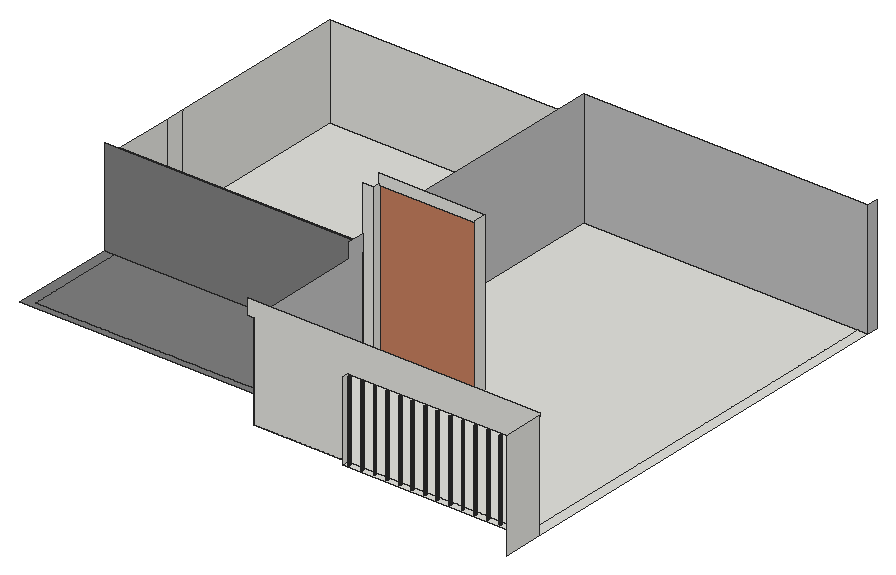
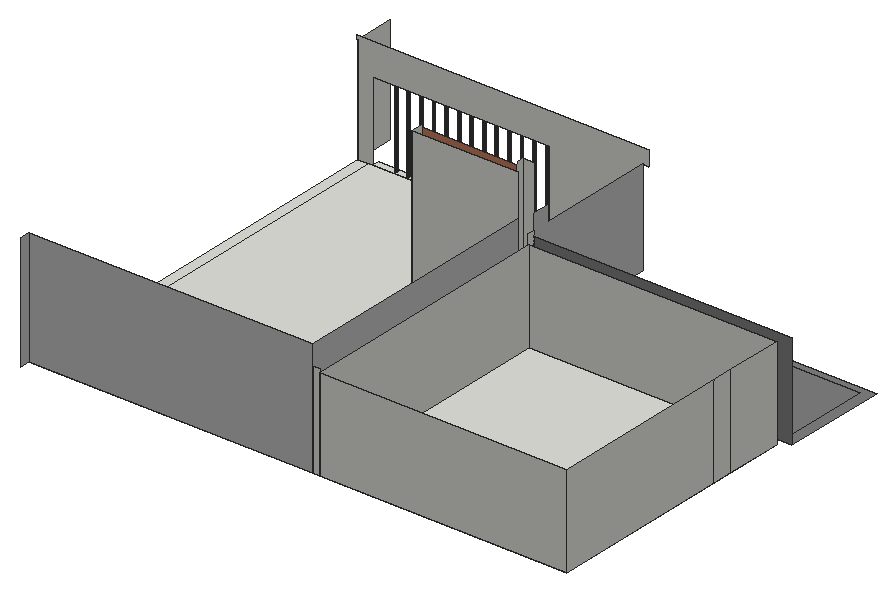
# SketchUp Ruby script. Lengths in inches.
U = 1.inch
M = Sketchup.active_model
def pt(a) = Geom::Point3d.new(a.map { |v| v * U })
def face(e, loops, mat)
  f = e.add_face(loops[0].map { |a| pt(a) })
  loops[1..].each { |l| e.add_face(l.map { |a| pt(a) }).erase! }
  f.material = f.back_material = mat if mat
  f
end
# faces: each face lists its corners as indices into pts; further lists are holes
def faces(e, pts, list, mat = nil) = list.each { |f| face(e, (f[0].is_a?(Array) ? f : [f]).map { |l| l.map { |i| pts[i] } }, mat) }
# xy, xz, yz: faces in a plane at the given z, y or x. An outline is a flat list of corners, or four numbers for a rectangle; further outlines are holes
def ring(l) = l.size == 4 ? [[l[0], l[1]], [l[2], l[1]], [l[2], l[3]], [l[0], l[3]]] : l.each_slice(2).to_a
def flat(e, list, mat, &to3) = list.each { |f| face(e, (f[0].is_a?(Array) ? f : [f]).map { |l| ring(l).map { |u, v| to3.(u, v) } }, mat) }
def xy(e, z, list, mat = nil) = flat(e, list, mat) { |x, y| [x, y, z] }
def xz(e, y, list, mat = nil) = flat(e, list, mat) { |x, z| [x, y, z] }
def yz(e, x, list, mat = nil) = flat(e, list, mat) { |y, z| [x, y, z] }
def lines(e, pts, list) = list.each { |a, b| e.add_line(pt(pts[a]), pt(pts[b])) }
# prism: a flat outline (further loops are holes) pulled along v
def prism(e, loops, v, mat = nil)
  f = face(e, loops, mat); d = Geom::Vector3d.new(v.map { |x| x * U })
  f.pushpull(f.normal.samedirection?(d) ? d.length : -d.length)
end
def box(e, o, s, mat = nil) = prism(e, [[o, [o[0] + s[0], o[1], o[2]], [o[0] + s[0], o[1] + s[1], o[2]], [o[0], o[1] + s[1], o[2]]]], [0, 0, s[2]], mat)
def at(x, y, z, deg = 0) = Geom::Transformation.translation(pt([x, y, z])) * Geom::Transformation.rotation(ORIGIN, Z_AXIS, deg.degrees)
def axes(o, x, y, z) = Geom::Transformation.new([*x, 0, *y, 0, *z, 0, *pt(o).to_a, 1])
def part(name) = M.definitions.add(name)
# library, detail: a bought-in or finely detailed component or shape, given as its bounding box
def library(name, o, s) = part(name).tap { |d| box(d.entities, o, s) }
def detail(e, o, s) = box(e.add_group.entities, o, s)
def put(e, d, t, mat = nil) = e.add_instance(d, t).tap { |i| i.material = mat if mat }
def group(e, t, mat = nil) = e.add_group.tap { |g| g.transformation = t; g.material = mat if mat }.entities
root = M.entities
M.materials.add("[0131_Silver]").color = [192, 192, 192]
M.materials.add("[0133_Gray]").color = [128, 128, 128]
M.materials.add("[0136_Charcoal]").color = [35, 35, 35]
M.materials.add("[Cladding Siding Tan]").color = [197, 126, 95]
xy(root,410,[[[329.48,44.6875,482.9375,50.6875],[333.11,46.6875,332.91,46.71,332.71,46.77,332.53,46.88,332.37,47.02,332.25,47.1875,332.16,47.38,332.12,47.58,332.12,47.79,332.16,48,332.25,48.1875,332.37,48.36,332.53,48.5,332.71,48.6,332.91,48.67,333.11,48.6875,333.32,48.67,333.52,48.6,333.7,48.5,333.86,48.36,333.98,48.1875,334.0625,48,334.11,47.79,334.11,47.58,334.0625,47.38,333.98,47.1875,333.86,47.02,333.7,46.88,333.52,46.77,333.32,46.71]],[333.11,46.6875,332.91,46.71,332.71,46.77,332.53,46.88,332.37,47.02,332.25,47.1875,332.16,47.38,332.12,47.58,332.12,47.79,332.16,48,332.25,48.1875,332.37,48.36,332.53,48.5,332.71,48.6,332.91,48.67,333.11,48.6875,333.32,48.67,333.52,48.6,333.7,48.5,333.86,48.36,333.98,48.1875,334.0625,48,334.11,47.79,334.11,47.58,334.0625,47.38,333.98,47.1875,333.86,47.02,333.7,46.88,333.52,46.77,333.32,46.71],[247.25,50.6875,486.875,50.6875,486.875,411,247.25,411,247.25,187,339.9375,187,339.9375,176.25,256.62,176.25,256.62,169.5,247.25,169.5],[486.875,50.6875,495.875,411],[247.25,169.5,256.62,176.25],
  [24.875,182.25,241.25,411]])
xy(root,410,[[15.875,84.25,241.25,84.25,241.25,90.25,24.875,90.25,24.875,176.25,15.875,176.25],[24.875,90.25,241.25,176.25]],"[0133_Gray]")
xz(root,50.6875,[[247.25,410,247.25,494,241.25,494,241.25,506.875,497.375,506.875,497.375,503.875,495.875,503.875,495.875,410,482.9375,410,482.9375,479,329.48,479,329.48,410]])
xz(root,169.5,[[247.25,410,256.62,547.1875]])
xz(root,176.25,[[15.875,410,241.25,494]],"[0133_Gray]")
xz(root,176.25,[[256.62,410,339.9375,545.23]],"[Cladding Siding Tan]")
xz(root,182.25,[[24.875,410,241.25,490.625]])
xz(root,187,[[247.25,410,339.9375,547.1875]])
xz(root,411,[[24.875,410,241.25,490.625],[241.25,410,247.25,494]])
xz(root,411,[[247.25,410,495.875,511]],"[0131_Silver]")
yz(root,24.875,[[182.25,410,233.22,490.625],[233.22,410,250.625,490.625],[250.625,410,411,490.625]])
yz(root,241.25,[[182.25,410,411,490.625]])
yz(root,247.25,[[169.5,410,176.25,494]])
yz(root,247.25,[[50.6875,410,169.5,410,169.5,507.4375,154.25,507.4375,154.25,494,50.6875,494],[187,410,411,511]],"[0131_Silver]")
yz(root,256.62,[[169.5,410,176.25,410,176.25,545.23,175.6875,545.23,175.6875,547.1875,169.5,547.1875]])
yz(root,329.48,[[44.6875,410,50.6875,479]])
yz(root,332.12,[[47.58,410,47.79,479]],"[0136_Charcoal]")
yz(root,334.11,[[47.58,410,47.79,479]],"[0136_Charcoal]")
yz(root,339.9375,[[176.25,410,187,410,187,547.1875,175.6875,547.1875,175.6875,545.23,176.25,545.23]])
yz(root,343.12,[[47.58,410,47.79,479]],"[0136_Charcoal]")
yz(root,345.11,[[47.58,410,47.79,479]],"[0136_Charcoal]")
yz(root,354.12,[[47.58,410,47.79,479]],"[0136_Charcoal]")
yz(root,356.11,[[47.58,410,47.79,479]],"[0136_Charcoal]")
yz(root,365.12,[[47.58,410,47.79,479]],"[0136_Charcoal]")
yz(root,367.11,[[47.58,410,47.79,479]],"[0136_Charcoal]")
yz(root,376.12,[[47.58,410,47.79,479]],"[0136_Charcoal]")
yz(root,378.11,[[47.58,410,47.79,479]],"[0136_Charcoal]")
yz(root,387.12,[[47.58,410,47.79,479]],"[0136_Charcoal]")
yz(root,389.11,[[47.58,410,47.79,479]],"[0136_Charcoal]")
yz(root,398.12,[[47.58,410,47.79,479]],"[0136_Charcoal]")
yz(root,400.11,[[47.58,410,47.79,479]],"[0136_Charcoal]")
yz(root,409.12,[[47.58,410,47.79,479]],"[0136_Charcoal]")
yz(root,411.11,[[47.58,410,47.79,479]],"[0136_Charcoal]")
yz(root,420.12,[[47.58,410,47.79,479]],"[0136_Charcoal]")
yz(root,422.11,[[47.58,410,47.79,479]],"[0136_Charcoal]")
yz(root,431.12,[[47.58,410,47.79,479]],"[0136_Charcoal]")
yz(root,433.11,[[47.58,410,47.79,479]],"[0136_Charcoal]")
yz(root,442.12,[[47.58,410,47.79,479]],"[0136_Charcoal]")
yz(root,444.11,[[47.58,410,47.79,479]],"[0136_Charcoal]")
yz(root,453.12,[[47.58,410,47.79,479]],"[0136_Charcoal]")
yz(root,455.11,[[47.58,410,47.79,479]],"[0136_Charcoal]")
yz(root,464.12,[[47.58,410,47.79,479]],"[0136_Charcoal]")
yz(root,466.11,[[47.58,410,47.79,479]],"[0136_Charcoal]")
yz(root,495.875,[[15.6875,410,50.6875,503.875]])
yz(root,495.875,[[411,410,420,511]],"[0131_Silver]")
p = [[332.71,46.77,410],[332.91,46.71,410],[332.91,46.71,479],[332.71,46.77,479],[333.11,46.6875,410],[333.11,46.6875,479],
  [333.32,46.71,410],[333.32,46.71,479],[333.52,46.77,410],[333.52,46.77,479],[343.71,46.77,410],[343.91,46.71,410],
  [343.91,46.71,479],[343.71,46.77,479],[344.11,46.6875,410],[344.11,46.6875,479],[344.32,46.71,410],[344.32,46.71,479],
  [344.52,46.77,410],[344.52,46.77,479],[354.71,46.77,410],[354.91,46.71,410],[354.91,46.71,479],[354.71,46.77,479],
  [355.11,46.6875,410],[355.11,46.6875,479],[355.32,46.71,410],[355.32,46.71,479],[355.52,46.77,410],[355.52,46.77,479],
  [365.71,46.77,410],[365.91,46.71,410],[365.91,46.71,479],[365.71,46.77,479],[366.11,46.6875,410],[366.11,46.6875,479],
  [366.32,46.71,410],[366.32,46.71,479],[366.52,46.77,410],[366.52,46.77,479],[376.71,46.77,410],[376.91,46.71,410],
  [376.91,46.71,479],[376.71,46.77,479],[377.11,46.6875,410],[377.11,46.6875,479],[377.32,46.71,410],[377.32,46.71,479],
  [377.52,46.77,410],[377.52,46.77,479],[387.71,46.77,410],[387.91,46.71,410],[387.91,46.71,479],[387.71,46.77,479],
  [388.11,46.6875,410],[388.11,46.6875,479],[388.32,46.71,410],[388.32,46.71,479],[388.52,46.77,410],[388.52,46.77,479],
  [398.71,46.77,410],[398.91,46.71,410],[398.91,46.71,479],[398.71,46.77,479],[399.11,46.6875,410],[399.11,46.6875,479],
  [399.32,46.71,410],[399.32,46.71,479],[399.52,46.77,410],[399.52,46.77,479],[409.71,46.77,410],[409.91,46.71,410],
  [409.91,46.71,479],[409.71,46.77,479],[410.11,46.6875,410],[410.11,46.6875,479],[410.32,46.71,410],[410.32,46.71,479],
  [410.52,46.77,410],[410.52,46.77,479],[420.71,46.77,410],[420.91,46.71,410],[420.91,46.71,479],[420.71,46.77,479],
  [421.11,46.6875,410],[421.11,46.6875,479],[421.32,46.71,410],[421.32,46.71,479],[421.52,46.77,410],[421.52,46.77,479],
  [431.71,46.77,410],[431.91,46.71,410],[431.91,46.71,479],[431.71,46.77,479],[432.11,46.6875,410],[432.11,46.6875,479],
  [432.32,46.71,410],[432.32,46.71,479],[432.52,46.77,410],[432.52,46.77,479],[442.71,46.77,410],[442.91,46.71,410],
  [442.91,46.71,479],[442.71,46.77,479],[443.11,46.6875,410],[443.11,46.6875,479],[443.32,46.71,410],[443.32,46.71,479],
  [443.52,46.77,410],[443.52,46.77,479],[453.71,46.77,410],[453.91,46.71,410],[453.91,46.71,479],[453.71,46.77,479],
  [454.11,46.6875,410],[454.11,46.6875,479],[454.32,46.71,410],[454.32,46.71,479],[454.52,46.77,410],[454.52,46.77,479],
  [464.71,46.77,410],[464.91,46.71,410],[464.91,46.71,479],[464.71,46.77,479],[465.11,46.6875,410],[465.11,46.6875,479],
  [465.32,46.71,410],[465.32,46.71,479],[465.52,46.77,410],[465.52,46.77,479],[332.53,46.88,410],[332.53,46.88,479],
  [333.7,46.88,410],[333.7,46.88,479],[343.53,46.88,410],[343.53,46.88,479],[344.7,46.88,410],[344.7,46.88,479],
  [354.53,46.88,410],[354.53,46.88,479],[355.7,46.88,410],[355.7,46.88,479],[365.53,46.88,410],[365.53,46.88,479],
  [366.7,46.88,410],[366.7,46.88,479],[376.53,46.88,410],[376.53,46.88,479],[377.7,46.88,410],[377.7,46.88,479],
  [387.53,46.88,410],[387.53,46.88,479],[388.7,46.88,410],[388.7,46.88,479],[398.53,46.88,410],[398.53,46.88,479],
  [399.7,46.88,410],[399.7,46.88,479],[409.53,46.88,410],[409.53,46.88,479],[410.7,46.88,410],[410.7,46.88,479],
  [420.53,46.88,410],[420.53,46.88,479],[421.7,46.88,410],[421.7,46.88,479],[431.53,46.88,410],[431.53,46.88,479],
  [432.7,46.88,410],[432.7,46.88,479],[442.53,46.88,410],[442.53,46.88,479],[443.7,46.88,410],[443.7,46.88,479],
  [453.53,46.88,410],[453.53,46.88,479],[454.7,46.88,410],[454.7,46.88,479],[464.53,46.88,410],[464.53,46.88,479],
  [465.7,46.88,410],[465.7,46.88,479],[332.37,47.02,410],[332.37,47.02,479],[333.86,47.02,410],[333.86,47.02,479],
  [343.37,47.02,410],[343.37,47.02,479],[344.86,47.02,410],[344.86,47.02,479],[354.37,47.02,410],[354.37,47.02,479],
  [355.86,47.02,410],[355.86,47.02,479],[365.37,47.02,410],[365.37,47.02,479],[366.86,47.02,410],[366.86,47.02,479],
  [376.37,47.02,410],[376.37,47.02,479],[377.86,47.02,410],[377.86,47.02,479],[387.37,47.02,410],[387.37,47.02,479],
  [388.86,47.02,410],[388.86,47.02,479],[398.37,47.02,410],[398.37,47.02,479],[399.86,47.02,410],[399.86,47.02,479],
  [409.37,47.02,410],[409.37,47.02,479],[410.86,47.02,410],[410.86,47.02,479],[420.37,47.02,410],[420.37,47.02,479],
  [421.86,47.02,410],[421.86,47.02,479],[431.37,47.02,410],[431.37,47.02,479],[432.86,47.02,410],[432.86,47.02,479],
  [442.37,47.02,410],[442.37,47.02,479],[443.86,47.02,410],[443.86,47.02,479],[453.37,47.02,410],[453.37,47.02,479],
  [454.86,47.02,410],[454.86,47.02,479],[464.37,47.02,410],[464.37,47.02,479],[465.86,47.02,410],[465.86,47.02,479],
  [332.25,47.1875,410],[332.25,47.1875,479],[333.98,47.1875,410],[333.98,47.1875,479],[343.25,47.1875,410],[343.25,47.1875,479],
  [344.98,47.1875,410],[344.98,47.1875,479],[354.25,47.1875,410],[354.25,47.1875,479],[355.98,47.1875,410],[355.98,47.1875,479],
  [365.25,47.1875,410],[365.25,47.1875,479],[366.98,47.1875,410],[366.98,47.1875,479],[376.25,47.1875,410],[376.25,47.1875,479],
  [377.98,47.1875,410],[377.98,47.1875,479],[387.25,47.1875,410],[387.25,47.1875,479],[388.98,47.1875,410],[388.98,47.1875,479],
  [398.25,47.1875,410],[398.25,47.1875,479],[399.98,47.1875,410],[399.98,47.1875,479],[409.25,47.1875,410],[409.25,47.1875,479],
  [410.98,47.1875,410],[410.98,47.1875,479],[420.25,47.1875,410],[420.25,47.1875,479],[421.98,47.1875,410],[421.98,47.1875,479],
  [431.25,47.1875,410],[431.25,47.1875,479],[432.98,47.1875,410],[432.98,47.1875,479],[442.25,47.1875,410],[442.25,47.1875,479],
  [443.98,47.1875,410],[443.98,47.1875,479],[453.25,47.1875,410],[453.25,47.1875,479],[454.98,47.1875,410],[454.98,47.1875,479],
  [464.25,47.1875,410],[464.25,47.1875,479],[465.98,47.1875,410],[465.98,47.1875,479],[332.16,47.38,410],[332.16,47.38,479],
  [334.0625,47.38,410],[334.0625,47.38,479],[343.16,47.38,410],[343.16,47.38,479],[345.0625,47.38,410],[345.0625,47.38,479],
  [354.16,47.38,410],[354.16,47.38,479],[356.0625,47.38,410],[356.0625,47.38,479],[365.16,47.38,410],[365.16,47.38,479],
  [367.0625,47.38,410],[367.0625,47.38,479],[376.16,47.38,410],[376.16,47.38,479],[378.0625,47.38,410],[378.0625,47.38,479],
  [387.16,47.38,410],[387.16,47.38,479],[389.0625,47.38,410],[389.0625,47.38,479],[398.16,47.38,410],[398.16,47.38,479],
  [400.0625,47.38,410],[400.0625,47.38,479],[409.16,47.38,410],[409.16,47.38,479],[411.0625,47.38,410],[411.0625,47.38,479],
  [420.16,47.38,410],[420.16,47.38,479],[422.0625,47.38,410],[422.0625,47.38,479],[431.16,47.38,410],[431.16,47.38,479],
  [433.0625,47.38,410],[433.0625,47.38,479],[442.16,47.38,410],[442.16,47.38,479],[444.0625,47.38,410],[444.0625,47.38,479],
  [453.16,47.38,410],[453.16,47.38,479],[455.0625,47.38,410],[455.0625,47.38,479],[464.16,47.38,410],[464.16,47.38,479],
  [466.0625,47.38,410],[466.0625,47.38,479],[332.12,47.58,410],[332.12,47.58,479],[334.11,47.58,410],[334.11,47.58,479],
  [343.12,47.58,410],[343.12,47.58,479],[345.11,47.58,410],[345.11,47.58,479],[354.12,47.58,410],[354.12,47.58,479],
  [356.11,47.58,410],[356.11,47.58,479],[365.12,47.58,410],[365.12,47.58,479],[367.11,47.58,410],[367.11,47.58,479],
  [376.12,47.58,410],[376.12,47.58,479],[378.11,47.58,410],[378.11,47.58,479],[387.12,47.58,410],[387.12,47.58,479],
  [389.11,47.58,410],[389.11,47.58,479],[398.12,47.58,410],[398.12,47.58,479],[400.11,47.58,410],[400.11,47.58,479],
  [409.12,47.58,410],[409.12,47.58,479],[411.11,47.58,410],[411.11,47.58,479],[420.12,47.58,410],[420.12,47.58,479],
  [422.11,47.58,410],[422.11,47.58,479],[431.12,47.58,410],[431.12,47.58,479],[433.11,47.58,410],[433.11,47.58,479],
  [442.12,47.58,410],[442.12,47.58,479],[444.11,47.58,410],[444.11,47.58,479],[453.12,47.58,410],[453.12,47.58,479],
  [455.11,47.58,410],[455.11,47.58,479],[464.12,47.58,410],[464.12,47.58,479],[466.11,47.58,410],[466.11,47.58,479],
  [332.16,48,410],[332.12,47.79,410],[332.12,47.79,479],[332.16,48,479],[334.11,47.79,410],[334.0625,48,410],
  [334.0625,48,479],[334.11,47.79,479],[343.16,48,410],[343.12,47.79,410],[343.12,47.79,479],[343.16,48,479],
  [345.11,47.79,410],[345.0625,48,410],[345.0625,48,479],[345.11,47.79,479],[354.16,48,410],[354.12,47.79,410],
  [354.12,47.79,479],[354.16,48,479],[356.11,47.79,410],[356.0625,48,410],[356.0625,48,479],[356.11,47.79,479],
  [365.16,48,410],[365.12,47.79,410],[365.12,47.79,479],[365.16,48,479],[367.11,47.79,410],[367.0625,48,410],
  [367.0625,48,479],[367.11,47.79,479],[376.16,48,410],[376.12,47.79,410],[376.12,47.79,479],[376.16,48,479],
  [378.11,47.79,410],[378.0625,48,410],[378.0625,48,479],[378.11,47.79,479],[387.16,48,410],[387.12,47.79,410],
  [387.12,47.79,479],[387.16,48,479],[389.11,47.79,410],[389.0625,48,410],[389.0625,48,479],[389.11,47.79,479],
  [398.16,48,410],[398.12,47.79,410],[398.12,47.79,479],[398.16,48,479],[400.11,47.79,410],[400.0625,48,410],
  [400.0625,48,479],[400.11,47.79,479],[409.16,48,410],[409.12,47.79,410],[409.12,47.79,479],[409.16,48,479],
  [411.11,47.79,410],[411.0625,48,410],[411.0625,48,479],[411.11,47.79,479],[420.16,48,410],[420.12,47.79,410],
  [420.12,47.79,479],[420.16,48,479],[422.11,47.79,410],[422.0625,48,410],[422.0625,48,479],[422.11,47.79,479],
  [431.16,48,410],[431.12,47.79,410],[431.12,47.79,479],[431.16,48,479],[433.11,47.79,410],[433.0625,48,410],
  [433.0625,48,479],[433.11,47.79,479],[442.16,48,410],[442.12,47.79,410],[442.12,47.79,479],[442.16,48,479],
  [444.11,47.79,410],[444.0625,48,410],[444.0625,48,479],[444.11,47.79,479],[453.16,48,410],[453.12,47.79,410],
  [453.12,47.79,479],[453.16,48,479],[455.11,47.79,410],[455.0625,48,410],[455.0625,48,479],[455.11,47.79,479],
  [464.16,48,410],[464.12,47.79,410],[464.12,47.79,479],[464.16,48,479],[466.11,47.79,410],[466.0625,48,410],
  [466.0625,48,479],[466.11,47.79,479],[332.25,48.1875,410],[332.25,48.1875,479],[333.98,48.1875,410],[333.98,48.1875,479],
  [343.25,48.1875,410],[343.25,48.1875,479],[344.98,48.1875,410],[344.98,48.1875,479],[354.25,48.1875,410],[354.25,48.1875,479],
  [355.98,48.1875,410],[355.98,48.1875,479],[365.25,48.1875,410],[365.25,48.1875,479],[366.98,48.1875,410],[366.98,48.1875,479],
  [376.25,48.1875,410],[376.25,48.1875,479],[377.98,48.1875,410],[377.98,48.1875,479],[387.25,48.1875,410],[387.25,48.1875,479],
  [388.98,48.1875,410],[388.98,48.1875,479],[398.25,48.1875,410],[398.25,48.1875,479],[399.98,48.1875,410],[399.98,48.1875,479],
  [409.25,48.1875,410],[409.25,48.1875,479],[410.98,48.1875,410],[410.98,48.1875,479],[420.25,48.1875,410],[420.25,48.1875,479],
  [421.98,48.1875,410],[421.98,48.1875,479],[431.25,48.1875,410],[431.25,48.1875,479],[432.98,48.1875,410],[432.98,48.1875,479],
  [442.25,48.1875,410],[442.25,48.1875,479],[443.98,48.1875,410],[443.98,48.1875,479],[453.25,48.1875,410],[453.25,48.1875,479],
  [454.98,48.1875,410],[454.98,48.1875,479],[464.25,48.1875,410],[464.25,48.1875,479],[465.98,48.1875,410],[465.98,48.1875,479],
  [332.37,48.36,410],[332.37,48.36,479],[333.86,48.36,410],[333.86,48.36,479],[343.37,48.36,410],[343.37,48.36,479],
  [344.86,48.36,410],[344.86,48.36,479],[354.37,48.36,410],[354.37,48.36,479],[355.86,48.36,410],[355.86,48.36,479],
  [365.37,48.36,410],[365.37,48.36,479],[366.86,48.36,410],[366.86,48.36,479],[376.37,48.36,410],[376.37,48.36,479],
  [377.86,48.36,410],[377.86,48.36,479],[387.37,48.36,410],[387.37,48.36,479],[388.86,48.36,410],[388.86,48.36,479],
  [398.37,48.36,410],[398.37,48.36,479],[399.86,48.36,410],[399.86,48.36,479],[409.37,48.36,410],[409.37,48.36,479],
  [410.86,48.36,410],[410.86,48.36,479],[420.37,48.36,410],[420.37,48.36,479],[421.86,48.36,410],[421.86,48.36,479],
  [431.37,48.36,410],[431.37,48.36,479],[432.86,48.36,410],[432.86,48.36,479],[442.37,48.36,410],[442.37,48.36,479],
  [443.86,48.36,410],[443.86,48.36,479],[453.37,48.36,410],[453.37,48.36,479],[454.86,48.36,410],[454.86,48.36,479],
  [464.37,48.36,410],[464.37,48.36,479],[465.86,48.36,410],[465.86,48.36,479],[332.53,48.5,410],[332.53,48.5,479],
  [333.7,48.5,410],[333.7,48.5,479],[343.53,48.5,410],[343.53,48.5,479],[344.7,48.5,410],[344.7,48.5,479],
  [354.53,48.5,410],[354.53,48.5,479],[355.7,48.5,410],[355.7,48.5,479],[365.53,48.5,410],[365.53,48.5,479],
  [366.7,48.5,410],[366.7,48.5,479],[376.53,48.5,410],[376.53,48.5,479],[377.7,48.5,410],[377.7,48.5,479],
  [387.53,48.5,410],[387.53,48.5,479],[388.7,48.5,410],[388.7,48.5,479],[398.53,48.5,410],[398.53,48.5,479],
  [399.7,48.5,410],[399.7,48.5,479],[409.53,48.5,410],[409.53,48.5,479],[410.7,48.5,410],[410.7,48.5,479],
  [420.53,48.5,410],[420.53,48.5,479],[421.7,48.5,410],[421.7,48.5,479],[431.53,48.5,410],[431.53,48.5,479],
  [432.7,48.5,410],[432.7,48.5,479],[442.53,48.5,410],[442.53,48.5,479],[443.7,48.5,410],[443.7,48.5,479],
  [453.53,48.5,410],[453.53,48.5,479],[454.7,48.5,410],[454.7,48.5,479],[464.53,48.5,410],[464.53,48.5,479],
  [465.7,48.5,410],[465.7,48.5,479],[332.71,48.6,410],[332.71,48.6,479],[333.52,48.6,410],[333.52,48.6,479],
  [343.71,48.6,410],[343.71,48.6,479],[344.52,48.6,410],[344.52,48.6,479],[354.71,48.6,410],[354.71,48.6,479],
  [355.52,48.6,410],[355.52,48.6,479],[365.71,48.6,410],[365.71,48.6,479],[366.52,48.6,410],[366.52,48.6,479],
  [376.71,48.6,410],[376.71,48.6,479],[377.52,48.6,410],[377.52,48.6,479],[387.71,48.6,410],[387.71,48.6,479],
  [388.52,48.6,410],[388.52,48.6,479],[398.71,48.6,410],[398.71,48.6,479],[399.52,48.6,410],[399.52,48.6,479],
  [409.71,48.6,410],[409.71,48.6,479],[410.52,48.6,410],[410.52,48.6,479],[420.71,48.6,410],[420.71,48.6,479],
  [421.52,48.6,410],[421.52,48.6,479],[431.71,48.6,410],[431.71,48.6,479],[432.52,48.6,410],[432.52,48.6,479],
  [442.71,48.6,410],[442.71,48.6,479],[443.52,48.6,410],[443.52,48.6,479],[453.71,48.6,410],[453.71,48.6,479],
  [454.52,48.6,410],[454.52,48.6,479],[464.71,48.6,410],[464.71,48.6,479],[465.52,48.6,410],[465.52,48.6,479],
  [332.91,48.67,410],[332.91,48.67,479],[333.32,48.67,410],[333.32,48.67,479],[343.91,48.67,410],[343.91,48.67,479],
  [344.32,48.67,410],[344.32,48.67,479],[354.91,48.67,410],[354.91,48.67,479],[355.32,48.67,410],[355.32,48.67,479],
  [365.91,48.67,410],[365.91,48.67,479],[366.32,48.67,410],[366.32,48.67,479],[376.91,48.67,410],[376.91,48.67,479],
  [377.32,48.67,410],[377.32,48.67,479],[387.91,48.67,410],[387.91,48.67,479],[388.32,48.67,410],[388.32,48.67,479],
  [398.91,48.67,410],[398.91,48.67,479],[399.32,48.67,410],[399.32,48.67,479],[409.91,48.67,410],[409.91,48.67,479],
  [410.32,48.67,410],[410.32,48.67,479],[420.91,48.67,410],[420.91,48.67,479],[421.32,48.67,410],[421.32,48.67,479],
  [431.91,48.67,410],[431.91,48.67,479],[432.32,48.67,410],[432.32,48.67,479],[442.91,48.67,410],[442.91,48.67,479],
  [443.32,48.67,410],[443.32,48.67,479],[453.91,48.67,410],[453.91,48.67,479],[454.32,48.67,410],[454.32,48.67,479],
  [464.91,48.67,410],[464.91,48.67,479],[465.32,48.67,410],[465.32,48.67,479],[333.11,48.6875,410],[333.11,48.6875,479],
  [344.11,48.6875,410],[344.11,48.6875,479],[355.11,48.6875,410],[355.11,48.6875,479],[366.11,48.6875,410],[366.11,48.6875,479],
  [377.11,48.6875,410],[377.11,48.6875,479],[388.11,48.6875,410],[388.11,48.6875,479],[399.11,48.6875,410],[399.11,48.6875,479],
  [410.11,48.6875,410],[410.11,48.6875,479],[421.11,48.6875,410],[421.11,48.6875,479],[432.11,48.6875,410],[432.11,48.6875,479],
  [443.11,48.6875,410],[443.11,48.6875,479],[454.11,48.6875,410],[454.11,48.6875,479],[465.11,48.6875,410],[465.11,48.6875,479]]
faces(root,p,[[0,1,2,3],[1,4,5,2],[4,6,7,5],[6,8,9,7],[10,11,12,13],[11,14,15,12],[14,16,17,15],[16,18,19,17],
  [20,21,22,23],[21,24,25,22],[24,26,27,25],[26,28,29,27],[30,31,32,33],[31,34,35,32],[34,36,37,35],[36,38,39,37],
  [40,41,42,43],[41,44,45,42],[44,46,47,45],[46,48,49,47],[50,51,52,53],[51,54,55,52],[54,56,57,55],[56,58,59,57],
  [60,61,62,63],[61,64,65,62],[64,66,67,65],[66,68,69,67],[70,71,72,73],[71,74,75,72],[74,76,77,75],[76,78,79,77],
  [80,81,82,83],[81,84,85,82],[84,86,87,85],[86,88,89,87],[90,91,92,93],[91,94,95,92],[94,96,97,95],[96,98,99,97],
  [100,101,102,103],[101,104,105,102],[104,106,107,105],[106,108,109,107],[110,111,112,113],[111,114,115,112],[114,116,117,115],[116,118,119,117],
  [120,121,122,123],[121,124,125,122],[124,126,127,125],[126,128,129,127],[130,0,3,131],[8,132,133,9],[134,10,13,135],[18,136,137,19],
  [138,20,23,139],[28,140,141,29],[142,30,33,143],[38,144,145,39],[146,40,43,147],[48,148,149,49],[150,50,53,151],[58,152,153,59],
  [154,60,63,155],[68,156,157,69],[158,70,73,159],[78,160,161,79],[162,80,83,163],[88,164,165,89],[166,90,93,167],[98,168,169,99],
  [170,100,103,171],[108,172,173,109],[174,110,113,175],[118,176,177,119],[178,120,123,179],[128,180,181,129],[182,130,131,183],[132,184,185,133],
  [186,134,135,187],[136,188,189,137],[190,138,139,191],[140,192,193,141],[194,142,143,195],[144,196,197,145],[198,146,147,199],[148,200,201,149],
  [202,150,151,203],[152,204,205,153],[206,154,155,207],[156,208,209,157],[210,158,159,211],[160,212,213,161],[214,162,163,215],[164,216,217,165],
  [218,166,167,219],[168,220,221,169],[222,170,171,223],[172,224,225,173],[226,174,175,227],[176,228,229,177],[230,178,179,231],[180,232,233,181],
  [234,182,183,235],[184,236,237,185],[238,186,187,239],[188,240,241,189],[242,190,191,243],[192,244,245,193],[246,194,195,247],[196,248,249,197],
  [250,198,199,251],[200,252,253,201],[254,202,203,255],[204,256,257,205],[258,206,207,259],[208,260,261,209],[262,210,211,263],[212,264,265,213],
  [266,214,215,267],[216,268,269,217],[270,218,219,271],[220,272,273,221],[274,222,223,275],[224,276,277,225],[278,226,227,279],[228,280,281,229],
  [282,230,231,283],[232,284,285,233],[286,234,235,287],[236,288,289,237],[290,238,239,291],[240,292,293,241],[294,242,243,295],[244,296,297,245],
  [298,246,247,299],[248,300,301,249],[302,250,251,303],[252,304,305,253],[306,254,255,307],[256,308,309,257],[310,258,259,311],[260,312,313,261],
  [314,262,263,315],[264,316,317,265],[318,266,267,319],[268,320,321,269],[322,270,271,323],[272,324,325,273],[326,274,275,327],[276,328,329,277],
  [330,278,279,331],[280,332,333,281],[334,282,283,335],[284,336,337,285],[338,286,287,339],[288,340,341,289],[342,290,291,343],[292,344,345,293],
  [346,294,295,347],[296,348,349,297],[350,298,299,351],[300,352,353,301],[354,302,303,355],[304,356,357,305],[358,306,307,359],[308,360,361,309],
  [362,310,311,363],[312,364,365,313],[366,314,315,367],[316,368,369,317],[370,318,319,371],[320,372,373,321],[374,322,323,375],[324,376,377,325],
  [378,326,327,379],[328,380,381,329],[382,330,331,383],[332,384,385,333],[386,334,335,387],[336,388,389,337],[390,391,392,393],[394,395,396,397],
  [398,399,400,401],[402,403,404,405],[406,407,408,409],[410,411,412,413],[414,415,416,417],[418,419,420,421],[422,423,424,425],[426,427,428,429],
  [430,431,432,433],[434,435,436,437],[438,439,440,441],[442,443,444,445],[446,447,448,449],[450,451,452,453],[454,455,456,457],[458,459,460,461],
  [462,463,464,465],[466,467,468,469],[470,471,472,473],[474,475,476,477],[478,479,480,481],[482,483,484,485],[486,487,488,489],[490,491,492,493],
  [494,390,393,495],[395,496,497,396],[498,398,401,499],[403,500,501,404],[502,406,409,503],[411,504,505,412],[506,414,417,507],[419,508,509,420],
  [510,422,425,511],[427,512,513,428],[514,430,433,515],[435,516,517,436],[518,438,441,519],[443,520,521,444],[522,446,449,523],[451,524,525,452],
  [526,454,457,527],[459,528,529,460],[530,462,465,531],[467,532,533,468],[534,470,473,535],[475,536,537,476],[538,478,481,539],[483,540,541,484],
  [542,486,489,543],[491,544,545,492],[546,494,495,547],[496,548,549,497],[550,498,499,551],[500,552,553,501],[554,502,503,555],[504,556,557,505],
  [558,506,507,559],[508,560,561,509],[562,510,511,563],[512,564,565,513],[566,514,515,567],[516,568,569,517],[570,518,519,571],[520,572,573,521],
  [574,522,523,575],[524,576,577,525],[578,526,527,579],[528,580,581,529],[582,530,531,583],[532,584,585,533],[586,534,535,587],[536,588,589,537],
  [590,538,539,591],[540,592,593,541],[594,542,543,595],[544,596,597,545],[598,546,547,599],[548,600,601,549],[602,550,551,603],[552,604,605,553],
  [606,554,555,607],[556,608,609,557],[610,558,559,611],[560,612,613,561],[614,562,563,615],[564,616,617,565],[618,566,567,619],[568,620,621,569],
  [622,570,571,623],[572,624,625,573],[626,574,575,627],[576,628,629,577],[630,578,579,631],[580,632,633,581],[634,582,583,635],[584,636,637,585],
  [638,586,587,639],[588,640,641,589],[642,590,591,643],[592,644,645,593],[646,594,595,647],[596,648,649,597],[650,598,599,651],[600,652,653,601],
  [654,602,603,655],[604,656,657,605],[658,606,607,659],[608,660,661,609],[662,610,611,663],[612,664,665,613],[666,614,615,667],[616,668,669,617],
  [670,618,619,671],[620,672,673,621],[674,622,623,675],[624,676,677,625],[678,626,627,679],[628,680,681,629],[682,630,631,683],[632,684,685,633],
  [686,634,635,687],[636,688,689,637],[690,638,639,691],[640,692,693,641],[694,642,643,695],[644,696,697,645],[698,646,647,699],[648,700,701,649],
  [702,650,651,703],[652,704,705,653],[706,654,655,707],[656,708,709,657],[710,658,659,711],[660,712,713,661],[714,662,663,715],[664,716,717,665],
  [718,666,667,719],[668,720,721,669],[722,670,671,723],[672,724,725,673],[726,674,675,727],[676,728,729,677],[730,678,679,731],[680,732,733,681],
  [734,682,683,735],[684,736,737,685],[738,686,687,739],[688,740,741,689],[742,690,691,743],[692,744,745,693],[746,694,695,747],[696,748,749,697],
  [750,698,699,751],[700,752,753,701],[754,702,703,755],[704,754,755,705],[756,706,707,757],[708,756,757,709],[758,710,711,759],[712,758,759,713],
  [760,714,715,761],[716,760,761,717],[762,718,719,763],[720,762,763,721],[764,722,723,765],[724,764,765,725],[766,726,727,767],[728,766,767,729],
  [768,730,731,769],[732,768,769,733],[770,734,735,771],[736,770,771,737],[772,738,739,773],[740,772,773,741],[774,742,743,775],[744,774,775,745],
  [776,746,747,777],[748,776,777,749],[778,750,751,779],[752,778,779,753]],"[0136_Charcoal]")
